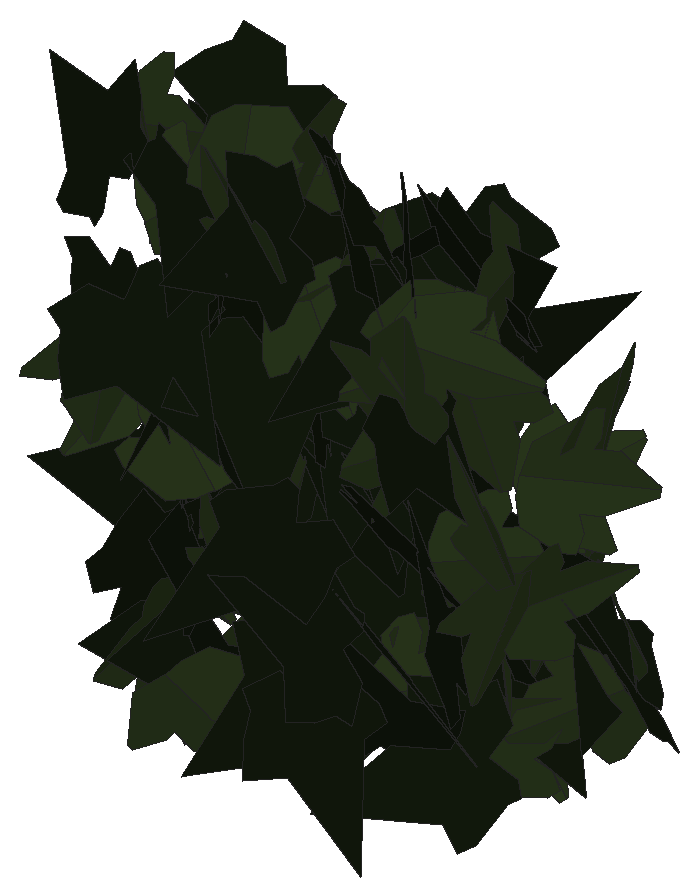
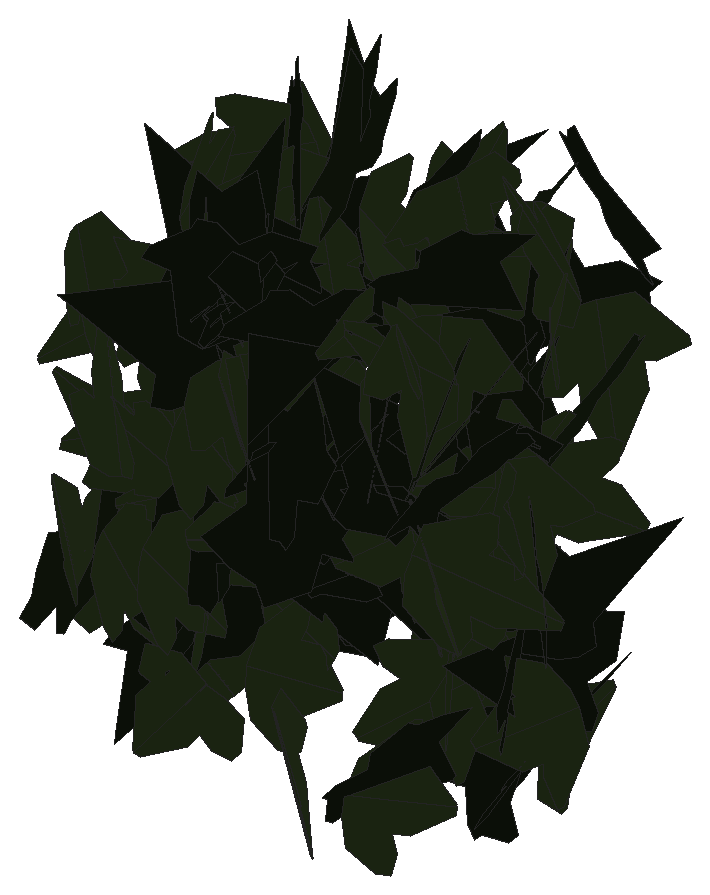
# SketchUp Ruby script. Lengths in inches.
U = 1.inch
M = Sketchup.active_model
def pt(a) = Geom::Point3d.new(a.map { |v| v * U })
def face(e, loops, mat)
  f = e.add_face(loops[0].map { |a| pt(a) })
  loops[1..].each { |l| e.add_face(l.map { |a| pt(a) }).erase! }
  f.material = f.back_material = mat if mat
  f
end
# faces: each face lists its corners as indices into pts; further lists are holes
def faces(e, pts, list, mat = nil) = list.each { |f| face(e, (f[0].is_a?(Array) ? f : [f]).map { |l| l.map { |i| pts[i] } }, mat) }
# xy, xz, yz: faces in a plane at the given z, y or x. An outline is a flat list of corners, or four numbers for a rectangle; further outlines are holes
def ring(l) = l.size == 4 ? [[l[0], l[1]], [l[2], l[1]], [l[2], l[3]], [l[0], l[3]]] : l.each_slice(2).to_a
def flat(e, list, mat, &to3) = list.each { |f| face(e, (f[0].is_a?(Array) ? f : [f]).map { |l| ring(l).map { |u, v| to3.(u, v) } }, mat) }
def xy(e, z, list, mat = nil) = flat(e, list, mat) { |x, y| [x, y, z] }
def xz(e, y, list, mat = nil) = flat(e, list, mat) { |x, z| [x, y, z] }
def yz(e, x, list, mat = nil) = flat(e, list, mat) { |y, z| [x, y, z] }
def lines(e, pts, list) = list.each { |a, b| e.add_line(pt(pts[a]), pt(pts[b])) }
# prism: a flat outline (further loops are holes) pulled along v
def prism(e, loops, v, mat = nil)
  f = face(e, loops, mat); d = Geom::Vector3d.new(v.map { |x| x * U })
  f.pushpull(f.normal.samedirection?(d) ? d.length : -d.length)
end
def box(e, o, s, mat = nil) = prism(e, [[o, [o[0] + s[0], o[1], o[2]], [o[0] + s[0], o[1] + s[1], o[2]], [o[0], o[1] + s[1], o[2]]]], [0, 0, s[2]], mat)
def at(x, y, z, deg = 0) = Geom::Transformation.translation(pt([x, y, z])) * Geom::Transformation.rotation(ORIGIN, Z_AXIS, deg.degrees)
def axes(o, x, y, z) = Geom::Transformation.new([*x, 0, *y, 0, *z, 0, *pt(o).to_a, 1])
def part(name) = M.definitions.add(name)
# library, detail: a bought-in or finely detailed component or shape, given as its bounding box
def library(name, o, s) = part(name).tap { |d| box(d.entities, o, s) }
def detail(e, o, s) = box(e.add_group.entities, o, s)
def put(e, d, t, mat = nil) = e.add_instance(d, t).tap { |i| i.material = mat if mat }
def group(e, t, mat = nil) = e.add_group.tap { |g| g.transformation = t; g.material = mat if mat }.entities
root = M.entities
M.materials.add("efeu1").color = [18, 25, 13]
M.materials.add("efeu2").color = [43, 57, 29]
c1 = part("ivyleaf_9")
p = [[1.54,2.16,1.25],[1.36,2.04,1.19],[-0.21,0.99,0.68],[-0.71,1.11,0.82],[-0.85,0.86,0.67],[-0.8,0.17,0.21],
  [-0.9,-0.01,0.1],[-0.67,-0.16,-0.02],[-0.08,-0.08,-0.05],[-0.03,-0.6,-0.4],[0.65,-0.88,-0.66],[0.83,-0.6,-0.49],
  [1.29,-0.42,-0.43],[1.8125,-0.07,-0.26],[1.21,0.44,0.15]]
faces(c1.entities,p,[[0,1,2,3,4,5,6,7,8,9,10,11,12,13,14]],"efeu1")
c2 = part("ivyleaf_10")
p = [[0,0.5,-0.03],[-0.0625,2.02,-0.43],[-0.19,2.01,-0.46],[-0.54,1.05,-0.29],[-0.52,0.625,-0.18],[-0.83,0.76,-0.28],
  [-1.16,0.64,-0.33],[-1.15,0.33,-0.24],[-0.77,-0.39,0.02],[-0.3,-0.51,0.16],[0.04,-0.48,0.23],[-0.02,2.01,-0.4375],
  [-0.06,2.01,-0.43],[0.04,-0.49,0.23],[0.67,-0.49,0.14],[1.38,0.36,-0.2],[1.375,0.51,-0.24],[0.81,0.65,-0.19],
  [0.62,0.59,-0.15],[0.6,1.09,-0.28],[0.5,1.23,-0.31]]
faces(c2.entities,p,[[0,1,2,3,4,5,6,7,8,9,10],[11,12,0,13,14,15,16,17,18,19,20]],"efeu2")
put(root,c1,axes([29.52,221,204.9],[-0.01789,-0.00494,-0.49966],[0.02678,-0.49927,0.00398],[-0.49896,-0.02661,0.01813]))
put(root,c1,axes([29.77,221.28,203.78],[0.02785,-0.48815,-0.10455],[0.03493,-0.10255,0.48812],[-0.498,-0.03449,0.02839]))
put(root,c1,axes([29.46,221.3,203.17],[0.07597,-0.44642,-0.21198],[-0.04187,0.20789,-0.4528],[0.49242,0.08655,-0.0058]))
put(root,c1,axes([29.03,221.87,202.88],[-0.18485,-0.30063,0.35419],[-0.18862,-0.29979,-0.35291],[0.42456,-0.26409,-0.00258]))
put(root,c2,axes([27.17,221.61,205.5],[-0.23318,-0.44044,0.04052],[-0.01529,-0.03775,-0.49834],[0.44203,-0.23365,0.00414]))
put(root,c1,axes([27.42,221.56,205.94],[-0.07924,-0.28137,-0.40565],[0.20633,0.35437,-0.2861],[0.4485,-0.21274,0.05995]))
put(root,c1,axes([29.57,221.9,203.62],[0.37923,-0.28722,0.15393],[0.12647,-0.08795,-0.47568],[0.30032,0.39971,0.00594]))
put(root,c2,axes([29.9,221.93,205.78],[-0.48829,0.00911,0.10719],[0.10674,-0.0212,0.48801],[0.01344,0.49947,0.01876]))
put(root,c2,axes([27.84,221.76,202.51],[-0.31218,-0.26218,-0.28949],[0.23649,0.16805,-0.40722],[0.31083,-0.39118,0.01909]))
put(root,c2,axes([30.92,221.85,204.76],[-0.3502,0.21738,-0.28304],[-0.23776,0.15362,0.41216],[0.26615,0.42326,-0.00423]))
put(root,c1,axes([29.52,222.14,202.46],[0.40831,-0.00237,0.28857],[-0.28855,0.00356,0.40832],[-0.00399,-0.49998,0.00154]))
put(root,c1,axes([28.32,222.42,206.5],[-0.15007,-0.20153,0.43228],[-0.19178,-0.38942,-0.24813],[0.43669,-0.24028,0.03958]))
put(root,c1,axes([29.12,222.35,206.84],[0.03792,-0.18606,0.46254],[0.10017,-0.45157,-0.18986],[0.48839,0.10706,0.00303]))
put(root,c1,axes([28.32,222.18,205.53],[-0.19563,-0.4198,-0.1884],[0.07343,0.17362,-0.4631],[0.45424,-0.20886,-0.00628]))
put(root,c1,axes([27.42,222.44,206.59],[-0.02293,-0.40205,0.29635],[0.05121,-0.297,-0.39896],[0.49684,0.01206,0.0548]))
put(root,c1,axes([30.34,222.05,203.39],[0.06737,-0.37046,0.32897],[-0.00468,0.33151,0.37427],[-0.49542,-0.05351,0.0412]))
put(root,c1,axes([27.66,222.1875,205.5],[-0.36638,0.24787,-0.23307],[0.19622,-0.12588,-0.44232],[-0.27796,-0.41559,-0.00503]))
put(root,c1,axes([26.95,221.88,206.88],[-0.07646,0.17876,0.46065],[-0.25826,0.38294,-0.19147],[-0.42125,-0.26722,0.03378]))
put(root,c2,axes([30.05,222.01,206.32],[-0.13837,-0.06505,-0.47605],[0.46365,0.11185,-0.15006],[0.12602,-0.48297,0.02936]))
put(root,c1,axes([27.39,222.4,205.71],[-0.02412,-0.00687,0.49937],[0.20037,-0.45809,0.00338],[0.45746,0.20028,0.02485]))
put(root,c2,axes([28.17,222.22,206.38],[-0.4469,0.14109,-0.17429],[-0.17582,0.02073,0.46761],[0.13918,0.47923,0.03108]))
put(root,c2,axes([30.6875,222.35,204.1],[-0.04367,-0.48185,0.12615],[-0.00813,-0.12593,-0.48381],[0.49802,-0.04431,0.00316]))
put(root,c1,axes([29.84,222.08,205.65],[0.23063,-0.2876,-0.33778],[-0.19584,0.2756,-0.36837],[0.39807,0.30221,0.01448]))
put(root,c2,axes([26.87,222.64,202.36],[-0.04724,-0.00237,-0.49776],[-0.03224,-0.49893,0.00544],[-0.49672,0.03261,0.04698]))
put(root,c1,axes([30.3,222.46,202.43],[-0.42744,-0.05844,0.25274],[-0.25039,-0.03441,-0.43142],[0.06782,-0.49538,0.00015]))
put(root,c1,axes([29.27,222.6875,206.04],[0.05171,-0.12346,-0.48175],[0.1387,-0.46155,0.13317],[-0.47759,-0.1474,-0.01348]))
put(root,c1,axes([29.3,222.24,204.43],[0.47578,-0.14506,0.05094],[0.05005,-0.01051,-0.49738],[0.14537,0.47838,0.00452]))
put(root,c2,axes([27.51,222.35,204.22],[0.32457,0.31666,0.21067],[-0.15741,-0.14029,0.45337],[0.34624,-0.36062,0.00862]))
put(root,c1,axes([26.52,222.49,205.51],[0.23123,-0.44096,0.04572],[0.02318,-0.03947,-0.4979],[0.44272,0.23237,0.00219]))
put(root,c1,axes([27.74,222.49,204.29],[0.19766,-0.41124,0.20449],[-0.08682,0.18515,0.45627],[-0.45099,-0.21588,0.00178]))
put(root,c2,axes([29.84,222.52,206.27],[0.30266,0.31368,-0.24495],[-0.16992,-0.17643,-0.43589],[-0.35989,0.3471,-0.00019]))
put(root,c2,axes([29.72,222.78,205.75],[-0.05135,0.01838,0.49702],[-0.06644,-0.49543,0.01145],[0.4929,-0.06486,0.05332]))
put(root,c2,axes([29.27,222.79,204.77],[-0.08509,0.13802,0.47298],[0.16154,-0.44564,0.1591],[0.46547,0.17989,0.03125]))
put(root,c2,axes([26.75,222.71,204.71],[0.17555,0.25688,-0.3914],[-0.21616,-0.32632,-0.31111],[-0.41528,0.27845,-0.00352]))
put(root,c1,axes([29.72,222.26,206.95],[0.07539,0.02497,-0.49365],[-0.48022,0.12198,-0.06716],[0.11708,0.48425,0.04237]))
put(root,c1,axes([28.69,222.79,206.96],[0.33846,-0.14498,-0.33827],[0.30569,-0.14516,0.36808],[-0.20493,-0.45597,-0.00962]))
put(root,c1,axes([27.02,222.89,202.12],[0.18162,-0.40121,-0.23674],[0.09157,-0.21839,0.44036],[-0.45676,-0.20331,-0.00585]))
put(root,c1,axes([26.89,222.85,203.54],[-0.05709,-0.03774,0.49529],[-0.39547,-0.29822,-0.06831],[0.30057,-0.39955,0.0042]))
put(root,c2,axes([27.75,222.57,202.99],[-0.44567,0.19624,-0.11344],[-0.10567,0.0415,0.48694],[0.20053,0.45801,0.00448]))
put(root,c2,axes([28.53,222.51,205.94],[0.18778,0.44242,0.13786],[0.05782,0.12522,-0.4806],[-0.45978,0.19644,-0.00413]))
put(root,c2,axes([27.23,222.33,206.47],[0.10264,0.08679,-0.48159],[0.29282,0.38336,0.1315],[0.39207,-0.30904,0.02787]))
put(root,c2,axes([27.71,222.73,207.0625],[0.19543,0.44127,-0.13072],[-0.05085,-0.12045,-0.48261],[-0.45741,0.20192,-0.0022]))
put(root,c2,axes([28.09,222.49,202.99],[-0.34767,0.1903,0.30481],[-0.2718,0.13817,-0.39628],[-0.23506,-0.44124,0.00737]))
put(root,c1,axes([27.94,222.28,205.63],[0.06542,0.10997,0.48335],[0.25386,0.41132,-0.12794],[-0.42577,0.26214,-0.00202]))
put(root,c2,axes([26.58,222.87,206.76],[0.12946,-0.12227,-0.46722],[0.36978,-0.28604,0.17732],[-0.31065,-0.39145,0.01636]))
put(root,c1,axes([26.78,222.35,202.86],[0.04994,0.06483,0.49326],[0.33682,0.36044,-0.08147],[-0.36614,0.34041,-0.00767]))
put(root,c1,axes([26.95,223.05,202.85],[-0.02697,0.00269,0.49926],[-0.07532,-0.49429,-0.00141],[0.49356,-0.07529,0.02707]))
put(root,c2,axes([27.87,222.7,202.52],[-0.33019,0.0439,-0.37289],[0.36829,-0.05873,-0.33304],[-0.07304,-0.49459,0.00644]))
put(root,c2,axes([29.22,222.73,202.54],[0.24535,-0.06807,-0.43031],[0.42267,-0.08254,0.25405],[-0.10562,-0.48842,0.01704]))
put(root,c2,axes([26.5,223.01,206.35],[-0.0284,-0.04778,0.4969],[0.40313,-0.29574,-0.00539],[0.29442,0.40032,0.05532]))
put(root,c1,axes([27.62,222.7,201.8],[0.11751,-0.16067,0.45867],[-0.27086,0.37015,0.19906],[-0.40352,-0.29525,-0.00005]))
put(root,c1,axes([28.52,222.83,206.13],[-0.03809,-0.01224,-0.4984],[-0.4416,-0.23116,0.03942],[-0.23138,0.44319,0.0068]))
put(root,c2,axes([28.05,222.86,203.99],[0.29277,-0.38566,-0.12472],[-0.07535,0.09938,-0.4842],[0.39826,0.30231,0.00008]))
put(root,c2,axes([29.95,223.2,206.4],[-0.03599,0.05626,0.49552],[0.28147,-0.40782,0.06674],[0.41168,0.28375,-0.00231]))
put(root,c2,axes([29.92,222.8125,205.46],[-0.42044,-0.25464,-0.09159],[0.07782,0.04832,-0.49154],[0.25918,-0.42758,-0.001]))
put(root,c2,axes([30.6875,222.55,203.86],[0.07521,-0.11695,0.48028],[0.08184,0.48205,0.10456],[-0.48749,0.06289,0.09165]))
put(root,c1,axes([28.71,223.1,203.51],[-0.336,-0.34723,-0.1286],[0.08844,0.09337,-0.48318],[0.35956,-0.34744,-0.00133]))
put(root,c1,axes([28.125,223.13,203.89],[-0.39314,-0.26059,-0.16593],[0.13997,0.08915,-0.47166],[0.2754,-0.41731,0.00285]))
put(root,c1,axes([28.42,222.82,204.61],[0.00696,-0.23838,0.43946],[-0.00048,0.4395,0.23841],[-0.49995,-0.00374,0.00589]))
put(root,c2,axes([28.67,223.06,205.72],[-0.24373,-0.43644,0.01069],[0.01175,0.00568,0.49983],[-0.43641,0.2439,0.00749]))
put(root,c2,axes([29.08,223.36,202.55],[0.07096,-0.2509,0.42663],[0.09904,-0.41508,-0.26058],[0.48493,0.12149,-0.00921]))
put(root,c1,axes([29.03,223.04,203.58],[0.09372,-0.05106,0.48848],[-0.43597,0.22034,0.10668],[-0.22615,-0.44592,-0.00322]))
put(root,c2,axes([29.93,222.99,202.14],[-0.31828,-0.15284,0.35403],[0.32303,0.14503,0.35302],[-0.2106,0.45344,0.00642]))
put(root,c2,axes([30.82,222.6875,205.04],[0.05333,0.13092,0.4796],[0.09989,0.46969,-0.13932],[-0.48701,0.11067,0.02394]))
put(root,c2,axes([28.75,222.99,205.125],[-0.44135,0.02554,-0.23358],[0.23357,-0.00647,-0.44204],[-0.0256,-0.49931,-0.00622]))
put(root,c2,axes([26.47,223.09,202.97],[-0.29931,0.09373,-0.3894],[0.36694,-0.13066,-0.3135],[-0.16053,-0.47344,0.00943]))
put(root,c1,axes([29.1875,223.37,205.875],[-0.2192,-0.44375,0.07097],[-0.02705,-0.06579,-0.49491],[0.44858,-0.22081,0.00484]))
put(root,c2,axes([30.96,223.18,202.91],[-0.24421,-0.0964,0.42552],[-0.37396,-0.20495,-0.26105],[0.22475,-0.44576,0.028]))
put(root,c2,axes([28.01,223.35,206.95],[0.17804,-0.3531,0.30598],[0.12133,-0.28127,-0.39518],[0.4512,0.21496,-0.01447]))
put(root,c1,axes([27.87,223.09,205.125],[0.0912,-0.42644,-0.2446],[-0.01905,0.24552,-0.43515],[0.49124,0.08869,0.02854]))
put(root,c1,axes([27.14,222.75,205.67],[-0.06634,0.46557,-0.16984],[-0.02313,0.16826,0.47027],[0.49504,0.07025,-0.00079]))
put(root,c1,axes([26.45,223.33,204.49],[-0.07262,-0.04701,-0.49246],[0.48572,-0.10119,-0.06196],[-0.09384,-0.48739,0.06037]))
put(root,c1,axes([28.42,223.42,204.61],[-0.10503,-0.48455,0.06465],[-0.00688,-0.06466,-0.49575],[0.4888,-0.10503,0.00691]))
put(root,c1,axes([29.72,223.4375,203],[0.35812,-0.13296,-0.3226],[0.29985,-0.11913,0.38197],[-0.17843,-0.46705,-0.00559]))
put(root,c2,axes([29.69,222.92,203.86],[-0.05754,-0.02862,-0.49585],[0.38677,0.31059,-0.06281],[0.31161,-0.39079,-0.01361]))
put(root,c1,axes([28.72,223.45,204.79],[-0.07751,-0.49053,-0.05809],[0.01073,0.05711,-0.49661],[0.49384,-0.07823,0.00168]))
put(root,c2,axes([26.82,223.28,204.91],[-0.40486,-0.26049,0.13503],[-0.11041,-0.07793,-0.48139],[0.27184,-0.41961,0.00558]))
put(root,c2,axes([27.53,223.45,206.37],[0.13144,-0.43989,0.19804],[0.05634,-0.18986,-0.45911],[0.47911,0.143,-0.00034]))
put(root,c2,axes([29.53,223.48,206.07],[0.27665,-0.18919,0.37105],[0.29833,-0.22082,-0.33502],[0.29063,0.40675,-0.0093]))
put(root,c2,axes([29.66,223.54,203],[-0.10049,0.13496,-0.47084],[0.22372,-0.41493,-0.16668],[-0.43572,-0.24417,0.02301]))
put(root,c2,axes([27.96,222.95,206.29],[-0.07584,-0.17878,-0.46075],[0.20651,0.41203,-0.19387],[0.449,-0.21971,0.01134]))
put(root,c1,axes([27.09,223.17,205.25],[0.00409,-0.26714,-0.42263],[0.12564,0.40963,-0.25771],[0.48394,-0.10409,0.07047]))
put(root,c2,axes([26.91,223.32,203.95],[-0.20156,-0.01479,0.45733],[0.45447,0.0516,0.20197],[-0.05317,0.49711,-0.00736]))
put(root,c2,axes([30.91,223.36,205.64],[0.09875,-0.48818,-0.04396],[-0.00988,0.04286,-0.49806],[0.49005,0.09923,-0.00118]))
put(root,c1,axes([29.44,223.49,206.06],[-0.01195,-0.09031,0.49163],[0.34728,-0.3552,-0.05681],[0.35952,0.34011,0.07122]))
put(root,c1,axes([30.67,223.7,203.25],[-0.02651,-0.41875,0.27193],[0.03352,-0.27319,-0.41742],[0.49817,-0.0039,0.04256]))
put(root,c1,axes([29.47,223.52,205.9],[0.36972,-0.28916,0.1723],[-0.1328,0.10988,0.46935],[-0.3093,-0.39282,0.00445]))
put(root,c1,axes([27.75,223.4,204.39],[0.27325,-0.19032,0.37297],[-0.29244,0.232,0.33264],[-0.29968,-0.39994,0.01548]))
put(root,c1,axes([27.3,223.67,206.9375],[-0.27959,-0.39827,0.11494],[-0.06163,-0.09716,-0.48658],[0.40992,-0.28625,0.00524]))
put(root,c1,axes([28.84,223.42,204.23],[-0.13979,0.16782,0.44977],[0.29489,-0.33963,0.21838],[0.37881,0.32633,-0.00402]))
put(root,c2,axes([26.89,223.07,204.86],[-0.00579,-0.18649,0.46388],[0.01308,0.4637,0.18658],[-0.4998,0.0143,-0.00049]))
put(root,c1,axes([27.71,223.61,204.63],[-0.49427,-0.07533,-0.00431],[0.00429,0.00051,-0.49998],[0.07533,-0.49429,0.00014]))
put(root,c2,axes([27.82,223.66,205.26],[0.30028,-0.28163,0.28375],[0.20204,-0.19932,-0.41164],[0.34498,0.36188,-0.0059]))
put(root,c1,axes([28.8125,223.14,206.08],[0.18129,0.45577,0.097],[0.03239,0.09151,-0.49049],[-0.46485,0.18413,0.00366]))
put(root,c2,axes([27.02,223.23,204.61],[0.01429,0.03794,-0.49835],[-0.33603,0.36979,0.01852],[0.36997,0.33439,0.03607]))
put(root,c1,axes([29.47,223.61,203.57],[0.1093,-0.08239,0.4809],[0.37111,-0.3059,-0.13675],[0.31675,0.38683,-0.00572]))
put(root,c1,axes([30.89,223.73,202.75],[0.29159,-0.40095,0.06495],[-0.03725,0.05321,0.49576],[-0.40446,-0.29396,0.00116]))
put(root,c1,axes([29.77,223.43,202.89],[0.00899,-0.35477,-0.35222],[-0.00098,0.35226,-0.35484],[0.49992,0.00707,0.00564]))
put(root,c1,axes([28.5,223.55,206.09],[-0.12365,-0.38758,-0.29068],[0.10292,0.27214,-0.40663],[0.47341,-0.16039,0.01248]))
put(root,c2,axes([29.17,223.57,205.16],[-0.39259,-0.27837,0.13559],[-0.10834,-0.08162,-0.48125],[0.29007,-0.40724,0.00377]))
put(root,c2,axes([27.625,223.92,202.17],[-0.00129,-0.19606,0.45995],[0.05354,-0.45736,-0.19481],[0.49712,0.04875,0.02218]))
put(root,c2,axes([30.68,223.77,203.14],[-0.16628,0.01315,0.47136],[0.42079,-0.22142,0.15461],[0.2128,0.44811,0.06257]))
put(root,c2,axes([29.4,223.8,204.79],[-0.03212,-0.42096,0.26788],[-0.01049,-0.26781,-0.4221],[0.49886,-0.03274,0.00837]))
put(root,c1,axes([27.41,223.71,204.94],[0.05609,-0.18047,0.46291],[0.39085,-0.27158,-0.15324],[0.30675,0.37904,0.11061]))
put(root,c1,axes([29.57,223.3,205.32],[0.06507,0.03766,0.49431],[0.45799,0.18628,-0.07448],[-0.18977,0.46247,-0.01025]))
put(root,c1,axes([29.2,223.62,206.42],[-0.16787,-0.31402,-0.35101],[0.16994,0.30715,-0.35606],[0.43925,-0.23885,0.00361]))
put(root,c2,axes([29.15,223.74,205.13],[0.31033,-0.38322,0.08269],[0.05285,-0.0636,-0.49311],[0.38846,0.3148,0.00104]))
put(root,c2,axes([27.24,223.57,206.1875],[-0.32397,-0.37392,-0.07228],[0.04736,0.05461,-0.49475],[0.37789,-0.32742,0.00004]))
put(root,c1,axes([26.625,223.91,205.99],[0.08841,-0.46344,0.16556],[0.02921,-0.16297,-0.47179],[0.49125,0.09309,-0.00174]))
put(root,c2,axes([28.81,223.6,203.95],[0.14459,0.03759,0.47716],[0.46312,0.11489,-0.14939],[-0.12087,0.48517,-0.0016]))
put(root,c2,axes([29.6875,223.93,203.54],[0.07484,-0.38391,0.31147],[0.0529,-0.30699,-0.3911],[0.49153,0.09149,-0.00534]))
put(root,c2,axes([27.42,223.68,204.58],[-0.30934,0.11691,-0.37502],[0.35351,-0.12529,-0.33066],[-0.17129,-0.46972,-0.00514]))
put(root,c2,axes([28.64,223.72,202.3],[0.28209,-0.41169,-0.03061],[-0.01378,0.02766,-0.49904],[0.41259,0.2824,0.00426]))
put(root,c1,axes([27.36,223.59,205.3],[0.01045,-0.33865,0.3677],[-0.02038,0.36719,0.33876],[-0.49947,-0.02207,-0.00613]))
put(root,c2,axes([27.17,223.77,206.08],[-0.01868,-0.05006,-0.49714],[0.46781,-0.1765,0.00019],[-0.1755,-0.46513,0.05343]))
put(root,c1,axes([26.81,223.85,205.34],[0.05263,-0.49279,-0.06622],[-0.00833,0.06571,-0.49559],[0.49715,0.05327,-0.0013]))
put(root,c1,axes([27.51,224.05,202.55],[-0.16691,-0.43159,0.1894],[-0.06969,-0.17612,-0.46274],[0.46614,-0.18087,-0.00136]))
put(root,c2,axes([29.57,223.68,202.32],[0.36489,0.09386,0.3287],[0.32105,0.07102,-0.37667],[-0.1174,0.48595,-0.00844]))
put(root,c2,axes([30.03,223.65,204.28],[0.30726,-0.02654,-0.39356],[0.39445,0.02138,0.30651],[0.00056,-0.49884,0.03407]))
put(root,c2,axes([30.13,223.92,203.48],[0.06407,-0.45722,0.19195],[0.01875,-0.19117,-0.46163],[0.49552,0.06635,-0.00735]))
put(root,c1,axes([28.37,223.95,204.67],[0.08631,-0.13089,0.47478],[0.27992,-0.38356,-0.15663],[0.40521,0.29284,0.00707]))
put(root,c1,axes([28.28,223.77,204.15],[0.42684,0.25198,0.06566],[-0.05676,-0.03302,0.49567],[0.25414,-0.4306,0.00041]))
put(root,c2,axes([30.1875,223.96,204.49],[0.08927,-0.41891,-0.25797],[0.09839,-0.24168,0.42651],[-0.48203,-0.12691,0.03929]))
put(root,c2,axes([26.9,223.95,204.48],[-0.12321,-0.08568,0.47695],[-0.36943,-0.30187,-0.14966],[0.31359,-0.38928,0.01109]))
put(root,c2,axes([26.98,223.8125,203.97],[0.37974,-0.30402,-0.11563],[0.09307,-0.06876,0.48643],[-0.31167,-0.39095,0.00436]))
